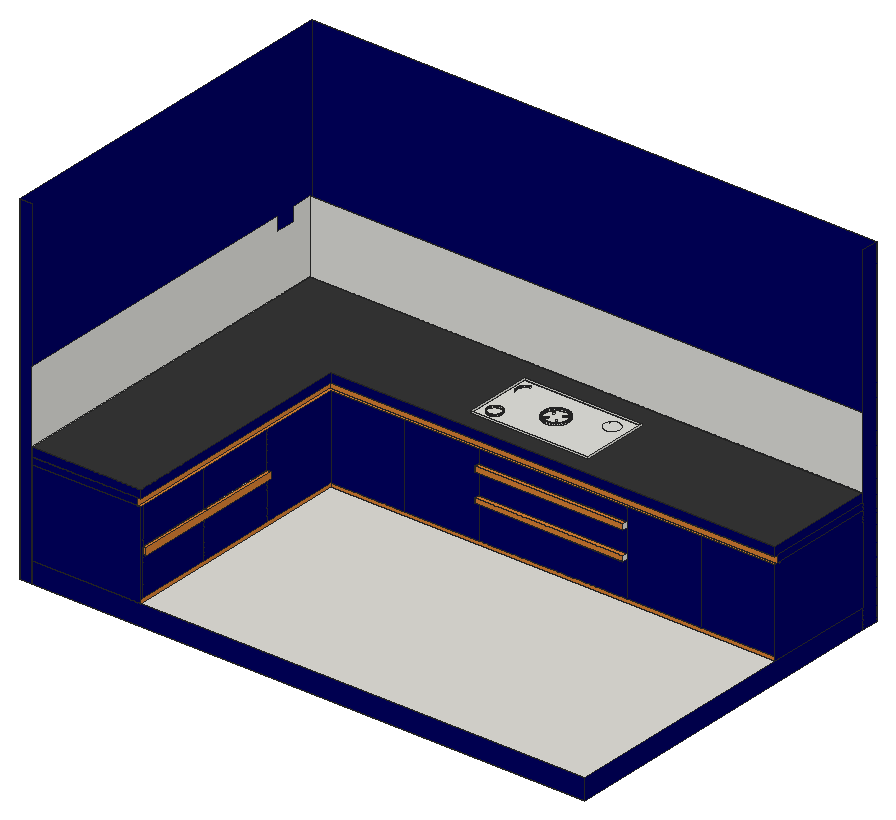
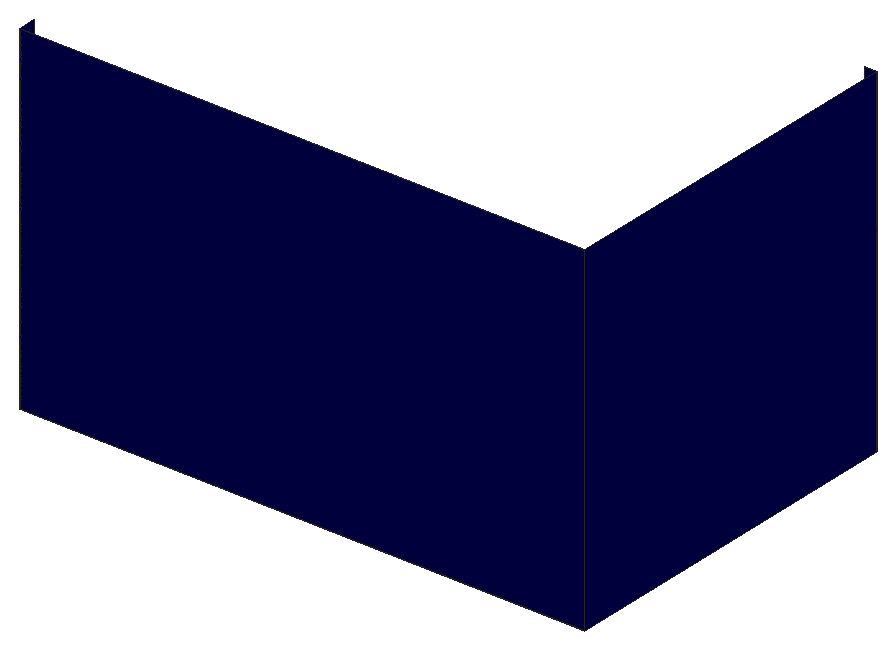
# SketchUp Ruby script. Lengths in inches.
U = 1.inch
M = Sketchup.active_model
def pt(a) = Geom::Point3d.new(a.map { |v| v * U })
def face(e, loops, mat)
  f = e.add_face(loops[0].map { |a| pt(a) })
  loops[1..].each { |l| e.add_face(l.map { |a| pt(a) }).erase! }
  f.material = f.back_material = mat if mat
  f
end
# faces: each face lists its corners as indices into pts; further lists are holes
def faces(e, pts, list, mat = nil) = list.each { |f| face(e, (f[0].is_a?(Array) ? f : [f]).map { |l| l.map { |i| pts[i] } }, mat) }
# xy, xz, yz: faces in a plane at the given z, y or x. An outline is a flat list of corners, or four numbers for a rectangle; further outlines are holes
def ring(l) = l.size == 4 ? [[l[0], l[1]], [l[2], l[1]], [l[2], l[3]], [l[0], l[3]]] : l.each_slice(2).to_a
def flat(e, list, mat, &to3) = list.each { |f| face(e, (f[0].is_a?(Array) ? f : [f]).map { |l| ring(l).map { |u, v| to3.(u, v) } }, mat) }
def xy(e, z, list, mat = nil) = flat(e, list, mat) { |x, y| [x, y, z] }
def xz(e, y, list, mat = nil) = flat(e, list, mat) { |x, z| [x, y, z] }
def yz(e, x, list, mat = nil) = flat(e, list, mat) { |y, z| [x, y, z] }
def lines(e, pts, list) = list.each { |a, b| e.add_line(pt(pts[a]), pt(pts[b])) }
# prism: a flat outline (further loops are holes) pulled along v
def prism(e, loops, v, mat = nil)
  f = face(e, loops, mat); d = Geom::Vector3d.new(v.map { |x| x * U })
  f.pushpull(f.normal.samedirection?(d) ? d.length : -d.length)
end
def box(e, o, s, mat = nil) = prism(e, [[o, [o[0] + s[0], o[1], o[2]], [o[0] + s[0], o[1] + s[1], o[2]], [o[0], o[1] + s[1], o[2]]]], [0, 0, s[2]], mat)
def at(x, y, z, deg = 0) = Geom::Transformation.translation(pt([x, y, z])) * Geom::Transformation.rotation(ORIGIN, Z_AXIS, deg.degrees)
def axes(o, x, y, z) = Geom::Transformation.new([*x, 0, *y, 0, *z, 0, *pt(o).to_a, 1])
def part(name) = M.definitions.add(name)
# library, detail: a bought-in or finely detailed component or shape, given as its bounding box
def library(name, o, s) = part(name).tap { |d| box(d.entities, o, s) }
def detail(e, o, s) = box(e.add_group.entities, o, s)
def put(e, d, t, mat = nil) = e.add_instance(d, t).tap { |i| i.material = mat if mat }
def group(e, t, mat = nil) = e.add_group.tap { |g| g.transformation = t; g.material = mat if mat }.entities
root = M.entities
M.materials.add("[0105_Navy]").color = [0, 0, 99]
M.materials.add("[Marble Carrara Gold Floor Tile]").color = [225, 223, 217]
M.materials.add("[Slate Light Tile]").color = [54, 54, 54]
M.materials.add("[Wood Bamboo]").color = [219, 130, 53]
xy(root,-49.625,[[0,0,0,887.375,1373.86,887.375,1373.86,845.75,28.58,845.75,28.58,0],[28.58,0,1373.86,845.75]])
xy(root,0,[[28.58,0,28.58,845.75,1373.86,845.75,1373.86,578.75,292.39,578.75,292.39,0]])
xy(root,0,[[292.39,0,1373.86,578.75]],"[Marble Carrara Gold Floor Tile]")
xy(root,96.15,[[652.88,567.25,1013.375,578.75]],"[Wood Bamboo]")
xy(root,104.9375,[[292.39,6.51,300.96,192.92],[292.39,192.92,300.96,385.83]],"[Wood Bamboo]")
xy(root,108.34,[[652.88,567.25,1013.375,578.75]],"[Wood Bamboo]")
xy(root,121.65,[[292.39,6.51,300.96,192.92],[292.39,192.92,300.96,385.83]],"[Wood Bamboo]")
xy(root,164.58,[[652.88,567.25,1013.375,578.75]],"[Wood Bamboo]")
xy(root,177.27,[[652.88,567.25,1013.375,578.75]],"[Wood Bamboo]")
xy(root,209.875,[[28.58,0,28.58,845.75,1373.86,845.75,1373.86,586.3125,284.83,586.3125,284.83,0]])
xy(root,209.875,[[284.83,0,284.83,586.3125,1373.86,586.3125,1373.86,578.75,292.39,578.75,292.39,0]],"[Wood Bamboo]")
xy(root,228.25,[[28.58,0,28.58,845.75,1373.86,845.75,1373.86,586.3125,284.83,586.3125,284.83,0]])
xy(root,228.25,[[284.83,0,292.39,578.75],[284.83,578.75,1373.86,586.3125]],"[Wood Bamboo]")
xy(root,248.9375,[[[28.58,0,292.39,0,292.39,578.75,1373.86,578.75,1373.86,845.75,28.58,845.75],[597.55,622.78,883.3,786.9]]],"[Slate Light Tile]")
xy(root,253.1875,[[739.6875,678.02,742.59,678.17,745.47,678.625,748.28,679.38,750.99,680.42,753.58,681.74,756.03,683.33,758.29,685.16,747.14,694.89,749.23,697.28,760.34,687.22,762.17,689.48,763.76,691.92,765.08,694.51,766.12,697.23,766.875,700.04,767.33,702.91,767.48,705.82,767.33,708.72,766.875,711.6,766.12,714.41,765.08,717.12,763.76,719.71,762.17,722.15,760.34,724.42,759.31,725.44,749.23,714.24,747.07,716.18,757.05,727.28,757.16,727.39,756.03,728.3,753.58,729.89,750.99,731.21,748.28,732.25,745.47,733,742.59,733.46,739.6875,733.61,736.78,733.46,733.91,733,731.1,732.25,728.38,731.21,725.79,729.89,723.35,728.3,721.09,726.47,719.03,724.42,728.12,716.18,726.2,714.05,717.2,722.15,715.61,719.71,714.29,717.12,713.25,714.41,712.5,711.6,712.04,708.72,711.89,705.82,712.04,702.91,712.5,700.04,713.25,697.23,714.29,694.51,715.61,691.92,717.2,689.48,719.03,687.22,720.06,686.1875,729.65,696.84,731.81,694.89,722.22,684.24,723.35,683.33,725.79,681.74,728.38,680.42,731.1,679.38,733.91,678.625,736.78,678.17],[844.95,726.98,846.82,727.07,848.68,727.37,850.49,727.85,852.24,728.53,853.91,729.38,855.49,730.4,856.94,731.58,858.27,732.91,853.22,736.57,854.32,738.09,859.45,734.36,860.47,735.9375,861.32,737.61,862,739.36,862.48,741.17,862.77,743.02,862.875,744.9,862.77,746.77,862.48,748.625,862,750.4375,861.32,752.1875,860.47,753.86,859.45,755.43,858.27,756.89,854.32,752.51,852.93,753.76,856.94,758.22,855.49,759.4,853.91,760.42,852.24,761.27,850.49,761.94,848.68,762.43,846.82,762.72,844.95,762.82,843.08,762.72,841.23,762.43,839.41,761.94,837.66,761.27,835.99,760.42,834.42,759.4,832.96,758.22,831.63,756.89,830.45,755.43,834.48,752.51,833.38,750.99,829.43,753.86,828.58,752.1875,827.91,750.4375,827.42,748.625,827.13,746.77,827.03,744.9,827.13,743.02,827.42,741.17,827.91,739.36,828.58,737.61,829.43,735.9375,830.45,734.36,831.63,732.91,832.96,731.58,837.46,736.57,838.85,735.32,834.42,730.4,835.99,729.38,837.66,728.53,839.41,727.85,841.23,727.37,843.08,727.07]])
xz(root,0,[[0,-49.625,28.58,779.8125],[28.58,-49.625,1373.86,0],[28.58,0,292.39,209.875],[28.58,209.875,284.83,228.25],[28.58,228.25,292.39,248.9375]],"[0105_Navy]")
xz(root,6.51,[[292.39,104.9375,300.96,121.65]],"[Wood Bamboo]")
xz(root,385.83,[[292.39,104.9375,300.96,121.65]])
xz(root,567.25,[[652.88,96.15,1013.375,108.34],[652.88,164.58,1013.375,177.27]],"[Wood Bamboo]")
xz(root,578.75,[[652.88,96.15,1013.375,108.34],[652.88,164.58,1013.375,177.27]])
xz(root,578.75,[[292.39,8.79,472.64,209.875],[472.64,8.79,652.88,209.875],[652.88,8.79,1013.375,96.15],[1013.375,8.79,1193.62,209.875],[1193.62,8.79,1373.86,209.875],
  [652.88,108.34,1013.375,164.58],[652.88,177.27,1013.375,209.875],[292.39,228.25,1373.86,248.9375]],"[0105_Navy]")
xz(root,578.75,[[292.39,0,1373.86,8.79]],"[Wood Bamboo]")
xz(root,586.3125,[[284.83,209.875,1373.86,228.25]],"[Wood Bamboo]")
xz(root,622.78,[[597.55,248.9375,883.3,253.1875]])
xz(root,786.9,[[597.55,248.9375,883.3,253.1875]])
xz(root,845.75,[[28.58,-49.625,1373.86,0],[28.58,0,1373.86,209.875],[28.58,209.875,1373.86,228.25],[28.58,228.25,1373.86,248.9375],[28.58,248.9375,1373.86,424.15]])
xz(root,887.375,[[0,-49.625,1373.86,779.8125]],"[0105_Navy]")
yz(root,0,[[0,-49.625,887.375,779.8125]],"[0105_Navy]")
yz(root,28.58,[[0,-49.625,845.75,0],[0,0,845.75,209.875],[0,209.875,845.75,228.25],[0,228.25,845.75,248.9375],[0,248.9375,845.75,248.9375,845.75,424.15,795.66,424.15,795.66,390.15,745.5625,390.15,745.5625,424.15,0,424.15]])
yz(root,284.83,[[0,209.875,586.3125,228.25]],"[Wood Bamboo]")
yz(root,292.39,[[6.51,104.9375,385.83,121.65]])
yz(root,292.39,[[0,8.79,6.51,209.875],[6.51,8.79,192.92,104.9375],[192.92,8.79,385.83,104.9375],[385.83,8.79,578.75,209.875],[6.51,121.65,192.92,209.875],
  [192.92,121.65,385.83,209.875],[0,228.25,578.75,248.9375]],"[0105_Navy]")
yz(root,292.39,[[0,0,578.75,8.79]],"[Wood Bamboo]")
yz(root,300.96,[[6.51,104.9375,385.83,121.65]],"[Wood Bamboo]")
yz(root,597.55,[[622.78,248.9375,786.9,253.1875]])
yz(root,652.88,[[567.25,96.15,578.75,108.34],[567.25,164.58,578.75,177.27]])
yz(root,883.3,[[622.78,248.9375,786.9,253.1875]])
yz(root,1013.375,[[567.25,96.15,578.75,108.34],[567.25,164.58,578.75,177.27]])
yz(root,1373.86,[[0,-49.625,845.75,0],[845.75,-49.625,887.375,779.8125],[578.75,0,845.75,209.875],[586.3125,209.875,845.75,228.25],[578.75,228.25,845.75,248.9375]],"[0105_Navy]")
p = [[634.4375,632.64,253.1875],[632.62,632.76,253.1875],[632.62,632.76,256.875],[634.4375,632.64,256.875],[636.26,632.71,253.1875],[636.26,632.71,256.875],
  [638.07,632.96,253.1875],[638.07,632.96,256.875],[630.82,633.08,253.1875],[630.82,633.08,256.875],[639.84,633.41,253.1875],[639.84,633.41,256.875],
  [629.07,633.58,253.1875],[629.07,633.58,256.875],[641.55,634.04,253.1875],[641.55,634.04,256.875],[627.38,634.26,253.1875],[627.38,634.26,256.875],
  [643.19,634.84,253.1875],[643.19,634.84,256.875],[625.77,635.11,253.1875],[625.77,635.11,256.875],[644.73,635.81,253.1875],[644.73,635.81,256.875],
  [624.25,636.125,253.1875],[624.25,636.125,256.875],[646.16,636.93,253.1875],[646.16,636.93,256.875],[622.85,637.29,253.1875],[622.85,637.29,255.75],
  [622.85,637.29,256.875],[647.47,638.2,253.1875],[647.47,638.2,256.875],[648.64,639.6,253.1875],[648.64,639.6,256.875],[621.58,638.6,253.1875],
  [620.46,640.04,253.1875],[620.46,640.04,256.875],[621.58,638.6,256.875],[621.58,638.6,255.75],[649.66,641.12,256.875],[649.66,641.12,255.75],
  [649.15,640.36,255.75],[649.15,640.36,253.1875],[619.49,641.58,253.1875],[619.49,641.58,256.875],[650.51,642.73,253.1875],[650.09,641.92,253.1875],
  [650.09,641.92,255.75],[650.51,642.73,256.875],[618.6875,643.22,253.1875],[618.6875,643.22,256.875],[651.19,644.42,253.1875],[651.19,644.42,256.875],
  [618.06,644.93,253.1875],[618.06,644.93,256.875],[651.69,646.17,253.1875],[651.69,646.17,256.875],[617.61,646.7,253.1875],[617.61,646.7,256.875],
  [652.01,647.97,253.1875],[652.01,647.97,256.875],[617.36,648.51,253.1875],[617.36,648.51,256.875],[652.13,649.79,253.1875],[652.13,649.79,256.875],
  [617.29,650.33,253.1875],[617.29,650.33,256.875],[652.0625,651.61,253.1875],[652.0625,651.61,256.875],[617.41,652.15,253.1875],[617.41,652.15,256.875],
  [651.8,653.42,253.1875],[651.8,653.42,256.875],[617.73,653.95,253.1875],[617.73,653.95,256.875],[651.36,655.18,253.1875],[651.36,655.18,256.875],
  [618.23,655.7,253.1875],[618.23,655.7,256.875],[650.73,656.9,253.1875],[650.73,656.9,256.875],[618.91,657.39,253.1875],[618.91,657.39,255.75],
  [618.91,657.39,256.875],[649.93,658.53,253.1875],[649.93,658.53,256.875],[648.96,660.08,253.1875],[648.96,660.08,256.875],[648.96,660.08,255.75],
  [619.76,659,253.1875],[620.78,660.52,253.1875],[620.78,660.52,256.875],[619.76,659,256.875],[619.76,659,255.75],[621.95,661.92,253.1875],
  [621.95,661.92,256.875],[646.57,662.82,253.1875],[647.84,661.51,253.1875],[647.84,661.51,255.75],[647.84,661.51,256.875],[646.57,662.82,256.875],
  [623.25,663.19,253.1875],[623.25,663.19,256.875],[645.17,663.99,253.1875],[645.17,663.99,256.875],[624.69,664.31,253.1875],[624.69,664.31,256.875],
  [643.65,665.01,253.1875],[643.65,665.01,256.875],[626.23,665.28,253.1875],[626.23,665.28,256.875],[642.04,665.86,253.1875],[642.04,665.86,256.875],
  [627.87,666.08,253.1875],[627.87,666.08,256.875],[640.35,666.54,253.1875],[640.35,666.54,256.875],[629.58,666.71,253.1875],[629.58,666.71,256.875],
  [638.6,667.04,253.1875],[638.6,667.04,256.875],[631.35,667.15,253.1875],[631.35,667.15,256.875],[636.8,667.35,253.1875],[636.8,667.35,256.875],
  [633.16,667.41,253.1875],[633.16,667.41,256.875],[634.98,667.48,253.1875],[634.98,667.48,256.875],[736.49,675.36,253.1875],[739.6875,675.19,253.1875],
  [739.6875,675.19,256.875],[736.49,675.36,256.875],[742.89,675.36,253.1875],[742.89,675.36,256.875],[733.32,675.86,253.1875],[733.32,675.86,256.875],
  [746.05,675.86,253.1875],[746.05,675.86,256.875],[730.22,676.69,253.1875],[730.22,676.69,256.875],[749.15,676.69,253.1875],[749.15,676.69,256.875],
  [727.23,677.84,253.1875],[727.23,677.84,256.875],[752.14,677.84,253.1875],[752.14,677.84,256.875],[724.375,679.29,253.1875],[724.375,679.29,256.875],
  [755,679.29,253.1875],[755,679.29,256.875],[739.6875,678.02,253.1875],[736.78,678.17,253.1875],[736.78,678.17,256.875],[739.6875,678.02,256.875],
  [742.59,678.17,253.1875],[742.59,678.17,256.875],[733.91,678.625,253.1875],[733.91,678.625,256.875],[745.47,678.625,253.1875],[745.47,678.625,256.875],
  [731.1,679.38,253.1875],[731.1,679.38,256.875],[748.28,679.38,253.1875],[748.28,679.38,256.875],[721.6875,681.04,253.1875],[721.6875,681.04,256.875],
  [757.6875,681.04,253.1875],[757.6875,681.04,256.875],[728.38,680.42,253.1875],[728.38,680.42,256.875],[750.99,680.42,253.1875],[750.99,680.42,256.875],
  [725.79,681.74,253.1875],[725.79,681.74,256.875],[753.58,681.74,253.1875],[753.58,681.74,256.875],[719.19,683.06,253.1875],[719.19,683.06,256.875],
  [760.18,683.06,253.1875],[760.18,683.06,256.875],[723.35,683.33,253.1875],[723.35,683.33,256.875],[756.03,683.33,253.1875],[756.03,683.33,256.875],
  [716.93,685.32,253.1875],[716.93,685.32,256.875],[762.45,685.32,253.1875],[762.45,685.32,256.875],[722.22,684.24,253.1875],[722.22,684.24,255.0625],
  [721.09,685.16,255.0625],[721.09,685.16,256.875],[758.29,685.16,253.1875],[758.29,685.16,256.875],[758.29,685.16,255.0625],[731.81,694.89,253.1875],
  [731.81,694.89,255.0625],[720.06,686.1875,255.0625],[720.06,686.1875,253.1875],[719.03,687.22,253.1875],[719.03,687.22,256.875],[747.14,694.89,253.1875],
  [747.14,694.89,255.0625],[714.91,687.82,253.1875],[714.91,687.82,256.875],[764.46,687.82,253.1875],[764.46,687.82,256.875],[729.65,696.84,253.1875],
  [729.65,696.84,255.0625],[717.2,689.48,253.1875],[717.2,689.48,256.875],[760.34,687.22,253.1875],[749.23,697.28,253.1875],[749.23,697.28,255.0625],
  [760.34,687.22,255.0625],[762.17,689.48,253.1875],[760.34,687.22,256.875],[762.17,689.48,256.875],[713.16,690.5,253.1875],[713.16,690.5,256.875],
  [766.21,690.5,253.1875],[766.21,690.5,256.875],[715.61,691.92,253.1875],[715.61,691.92,256.875],[763.76,691.92,253.1875],[763.76,691.92,256.875],
  [711.71,693.36,253.1875],[711.71,693.36,256.875],[767.66,693.36,253.1875],[767.66,693.36,256.875],[714.29,694.51,253.1875],[714.29,694.51,256.875],
  [765.08,694.51,253.1875],[765.08,694.51,256.875],[710.5625,696.35,253.1875],[710.5625,696.35,256.875],[768.8125,696.35,253.1875],[768.8125,696.35,256.875],
  [713.25,697.23,253.1875],[713.25,697.23,256.875],[766.12,697.23,253.1875],[766.12,697.23,256.875],[709.73,699.45,253.1875],[709.73,699.45,256.875],
  [769.64,699.45,253.1875],[769.64,699.45,256.875],[712.5,700.04,253.1875],[712.5,700.04,256.875],[766.875,700.04,253.1875],[766.875,700.04,256.875],
  [709.23,702.61,253.1875],[709.23,702.61,256.875],[770.14,702.61,253.1875],[770.14,702.61,256.875],[712.04,702.91,253.1875],[712.04,702.91,256.875],
  [767.33,702.91,253.1875],[767.33,702.91,256.875],[709.0625,705.82,253.1875],[709.0625,705.82,256.875],[770.3125,705.82,253.1875],[770.3125,705.82,256.875],
  [711.89,705.82,253.1875],[711.89,705.82,256.875],[767.48,705.82,253.1875],[767.48,705.82,256.875],[709.23,709.02,253.1875],[709.23,709.02,256.875],
  [712.04,708.72,253.1875],[712.04,708.72,256.875],[767.33,708.72,253.1875],[767.33,708.72,256.875],[770.14,709.02,253.1875],[770.14,709.02,256.875],
  [712.5,711.6,253.1875],[712.5,711.6,256.875],[766.875,711.6,253.1875],[766.875,711.6,256.875],[709.73,712.18,253.1875],[709.73,712.18,256.875],
  [769.64,712.18,253.1875],[769.64,712.18,256.875],[713.25,714.41,253.1875],[713.25,714.41,256.875],[766.12,714.41,253.1875],[766.12,714.41,256.875],
  [710.5625,715.28,253.1875],[710.5625,715.28,256.875],[768.8125,715.28,253.1875],[768.8125,715.28,256.875],[717.2,722.15,253.1875],[726.2,714.05,253.1875],
  [726.2,714.05,255.0625],[717.2,722.15,255.0625],[728.12,716.18,253.1875],[728.12,716.18,255.0625],[747.07,716.18,253.1875],[749.23,714.24,253.1875],
  [749.23,714.24,255.0625],[747.07,716.18,255.0625],[759.31,725.44,253.1875],[759.31,725.44,255.0625],[714.29,717.12,253.1875],[714.29,717.12,256.875],
  [765.08,717.12,253.1875],[765.08,717.12,256.875],[711.71,718.27,253.1875],[711.71,718.27,256.875],[767.66,718.27,253.1875],[767.66,718.27,256.875],
  [719.03,724.42,253.1875],[719.03,724.42,255.0625],[757.05,727.28,253.1875],[757.05,727.28,255.0625],[715.61,719.71,253.1875],[715.61,719.71,256.875],
  [763.76,719.71,253.1875],[763.76,719.71,256.875],[713.16,721.13,253.1875],[713.16,721.13,256.875],[766.21,721.13,253.1875],[766.21,721.13,256.875],
  [717.2,722.15,256.875],[762.17,722.15,253.1875],[762.17,722.15,256.875],[714.91,723.82,253.1875],[714.91,723.82,256.875],[764.46,723.82,253.1875],
  [764.46,723.82,256.875],[760.34,724.42,253.1875],[760.34,724.42,256.875],[716.93,726.31,253.1875],[716.93,726.31,256.875],[762.45,726.31,253.1875],
  [762.45,726.31,256.875],[721.09,726.47,253.1875],[721.09,726.47,256.875],[719.03,724.42,256.875],[758.29,726.47,256.875],[758.29,726.47,255.0625],
  [719.19,728.57,253.1875],[719.19,728.57,256.875],[760.18,728.57,253.1875],[760.18,728.57,256.875],[723.35,728.3,253.1875],[723.35,728.3,256.875],
  [756.03,728.3,253.1875],[757.16,727.39,253.1875],[757.16,727.39,255.0625],[756.03,728.3,256.875],[725.79,729.89,253.1875],[725.79,729.89,256.875],
  [753.58,729.89,253.1875],[753.58,729.89,256.875],[721.6875,730.59,253.1875],[721.6875,730.59,256.875],[757.6875,730.59,253.1875],[757.6875,730.59,256.875],
  [728.38,731.21,253.1875],[728.38,731.21,256.875],[750.99,731.21,253.1875],[750.99,731.21,256.875],[724.375,732.34,253.1875],[724.375,732.34,256.875],
  [755,732.34,253.1875],[755,732.34,256.875],[731.1,732.25,253.1875],[731.1,732.25,256.875],[748.28,732.25,253.1875],[748.28,732.25,256.875],
  [727.23,733.79,253.1875],[727.23,733.79,256.875],[733.91,733,253.1875],[733.91,733,256.875],[745.47,733,253.1875],[745.47,733,256.875],
  [752.14,733.79,253.1875],[752.14,733.79,256.875],[736.78,733.46,253.1875],[736.78,733.46,256.875],[742.59,733.46,253.1875],[742.59,733.46,256.875],
  [739.6875,733.61,253.1875],[739.6875,733.61,256.875],[730.22,734.94,253.1875],[730.22,734.94,256.875],[749.15,734.94,253.1875],[749.15,734.94,256.875],
  [616.16,734.1875,253.1875],[615.14,736.19,253.1875],[615.14,736.19,256.875],[616.16,734.1875,256.875],[733.32,735.77,253.1875],[733.32,735.77,256.875],
  [746.05,735.77,253.1875],[746.05,735.77,256.875],[736.49,736.27,253.1875],[736.49,736.27,256.875],[742.89,736.27,253.1875],[742.89,736.27,256.875],
  [614.34,738.28,253.1875],[614.34,738.28,256.875],[739.6875,736.44,253.1875],[739.6875,736.44,256.875],[613.76,740.44,253.1875],[613.76,740.44,256.875],
  [613.41,742.66,253.1875],[613.41,742.66,256.875],[613.29,744.9,253.1875],[613.29,744.9,256.875],[613.41,747.14,253.1875],[613.41,747.14,256.875],
  [613.76,749.35,253.1875],[613.76,749.35,256.875],[614.34,751.52,253.1875],[614.34,751.52,256.875],[615.14,753.61,253.1875],[615.14,753.61,256.875],
  [616.16,755.61,253.1875],[616.16,755.61,256.875],[617.38,757.49,253.1875],[617.38,757.49,255.1875],[617.38,757.49,256.875],[618.79,759.23,253.1875],
  [620.375,760.82,253.1875],[620.375,760.82,256.875],[618.79,759.23,256.875],[618.79,759.23,255.1875],[622.12,762.23,253.1875],[622.12,762.23,256.875],
  [624,763.45,253.1875],[624,763.45,256.875],[626,764.47,253.1875],[626,764.47,256.875],[628.09,765.27,253.1875],[628.09,765.27,256.875],
  [630.26,765.85,253.1875],[630.26,765.85,256.875],[759.42,725.56,253.1875],[719.96,686.07,253.1875]]
faces(root,p,[[0,1,2,3],[4,0,3,5],[6,4,5,7],[1,8,9,2],[10,6,7,11],[8,12,13,9],[14,10,11,15],[12,16,17,13],
  [18,14,15,19],[16,20,21,17],[22,18,19,23],[20,24,25,21],[26,22,23,27],[24,28,29,30,25],[31,26,27,32],[33,31,32,34],
  [35,36,37,38,39],[40,41,42,43,33,34],[36,44,45,37],[46,47,48,41,40,49],[44,50,51,45],[52,46,49,53],[50,54,55,51],[56,52,53,57],
  [54,58,59,55],[60,56,57,61],[58,62,63,59],[64,60,61,65],[62,66,67,63],[68,64,65,69],[66,70,71,67],[72,68,69,73],
  [70,74,75,71],[76,72,73,77],[74,78,79,75],[80,76,77,81],[78,82,83,84,79],[85,80,81,86],[87,85,86,88,89],[90,91,92,93,94],
  [91,95,96,92],[97,98,99,100,101],[95,102,103,96],[104,97,101,105],[102,106,107,103],[108,104,105,109],[106,110,111,107],[112,108,109,113],
  [110,114,115,111],[116,112,113,117],[114,118,119,115],[120,116,117,121],[118,122,123,119],[124,120,121,125],[122,126,127,123],[126,128,129,127],
  [128,124,125,129],[130,131,132,133],[131,134,135,132],[136,130,133,137],[134,138,139,135],[140,136,137,141],[138,142,143,139],[144,140,141,145],
  [142,146,147,143],[148,144,145,149],[146,150,151,147],[152,153,154,155],[156,152,155,157],[153,158,159,154],[160,156,157,161],[158,162,163,159],
  [164,160,161,165],[166,148,149,167],[150,168,169,151],[162,170,171,163],[172,164,165,173],[170,174,175,171],[176,172,173,177],[178,166,167,179],
  [168,180,181,169],[174,182,183,175],[184,176,177,185],[186,178,179,187],[180,188,189,181],[182,190,191,192,193,183],[194,184,185,195,196],[190,197,198,191],
  [193,192,199,200,201,202],[203,194,196,204],[205,186,187,206],[188,207,208,189],[209,200,199,210],[201,211,212,202],[213,214,215,216],[217,213,216,218,219],
  [220,205,206,221],[207,222,223,208],[211,224,225,212],[226,217,219,227],[228,220,221,229],[222,230,231,223],[224,232,233,225],[234,226,227,235],
  [236,228,229,237],[230,238,239,231],[232,240,241,233],[242,234,235,243],[197,209,210,198],[214,203,204,215],[244,236,237,245],[238,246,247,239],
  [240,248,249,241],[250,242,243,251],[252,244,245,253],[246,254,255,247],[248,256,257,249],[258,250,251,259],[260,252,253,261],[254,262,263,255],
  [256,264,265,257],[266,258,259,267],[268,260,261,269],[264,270,271,265],[272,266,267,273],[262,274,275,263],[270,276,277,271],[278,272,273,279],
  [280,268,269,281],[274,282,283,275],[276,284,285,277],[286,278,279,287],[288,280,281,289],[282,290,291,283],[292,293,294,295],[293,296,297,294],
  [298,299,300,301],[299,302,303,300],[284,304,305,285],[306,286,287,307],[308,288,289,309],[290,310,311,291],[296,312,313,297],[314,298,301,315],
  [304,316,317,305],[318,306,307,319],[320,308,309,321],[310,322,323,311],[316,292,295,324,317],[325,318,319,326],[327,320,321,328],[322,329,330,323],
  [331,325,326,332],[333,327,328,334],[329,335,336,330],[312,337,338,339,313],[340,341,303,302,331,332],[342,333,334,343],[335,344,345,336],[337,346,347,338],
  [348,349,350,341,340,351],[349,314,315,350],[346,352,353,347],[354,348,351,355],[356,342,343,357],[344,358,359,345],[352,360,361,353],[362,354,355,363],
  [364,356,357,365],[358,366,367,359],[360,368,369,361],[370,362,363,371],[372,364,365,373],[368,374,375,369],[376,370,371,377],[366,378,379,367],
  [374,380,381,375],[382,376,377,383],[380,384,385,381],[384,382,383,385],[386,372,373,387],[378,388,389,379],[390,391,392,393],[394,386,387,395],
  [388,396,397,389],[398,394,395,399],[396,400,401,397],[391,402,403,392],[404,398,399,405],[400,404,405,401],[402,406,407,403],[406,408,409,407],
  [408,410,411,409],[410,412,413,411],[412,414,415,413],[414,416,417,415],[416,418,419,417],[418,420,421,419],[420,422,423,424,421],[425,426,427,428,429],
  [426,430,431,427],[430,432,433,431],[432,434,435,433],[434,436,437,435],[436,438,439,437]])
lines(root,p,[[302,440],[200,441]])
